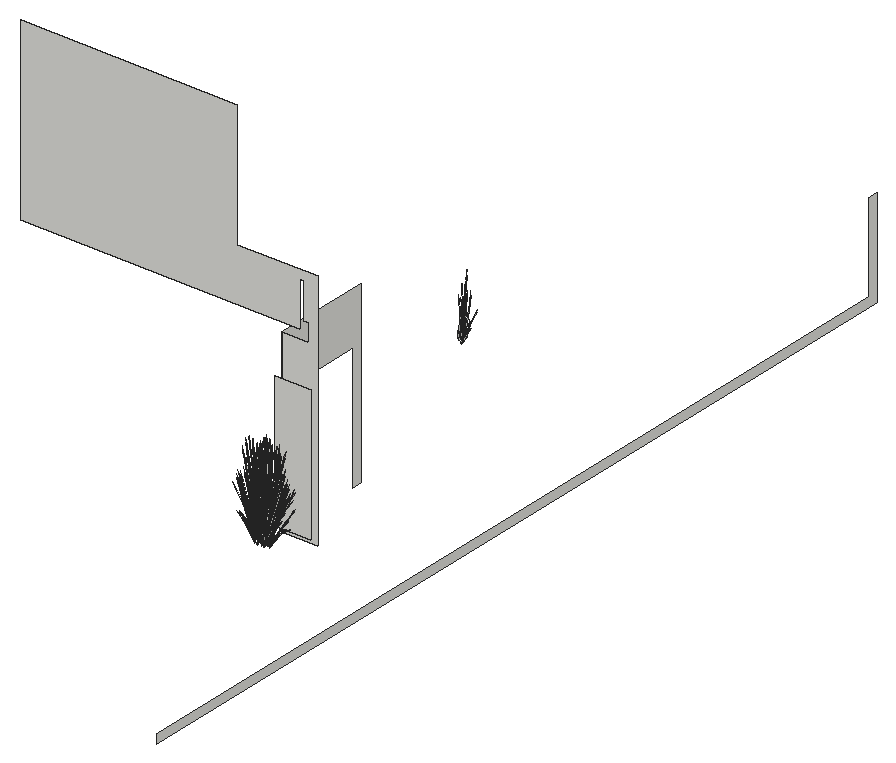
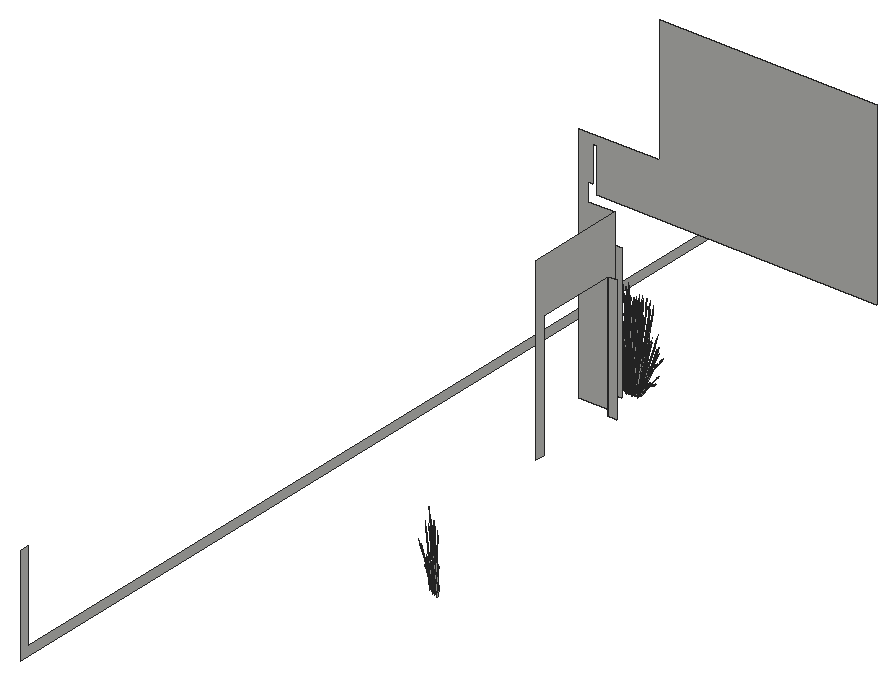
# SketchUp Ruby script. Lengths in inches.
U = 1.inch
M = Sketchup.active_model
def pt(a) = Geom::Point3d.new(a.map { |v| v * U })
def face(e, loops, mat)
  f = e.add_face(loops[0].map { |a| pt(a) })
  loops[1..].each { |l| e.add_face(l.map { |a| pt(a) }).erase! }
  f.material = f.back_material = mat if mat
  f
end
# faces: each face lists its corners as indices into pts; further lists are holes
def faces(e, pts, list, mat = nil) = list.each { |f| face(e, (f[0].is_a?(Array) ? f : [f]).map { |l| l.map { |i| pts[i] } }, mat) }
# xy, xz, yz: faces in a plane at the given z, y or x. An outline is a flat list of corners, or four numbers for a rectangle; further outlines are holes
def ring(l) = l.size == 4 ? [[l[0], l[1]], [l[2], l[1]], [l[2], l[3]], [l[0], l[3]]] : l.each_slice(2).to_a
def flat(e, list, mat, &to3) = list.each { |f| face(e, (f[0].is_a?(Array) ? f : [f]).map { |l| ring(l).map { |u, v| to3.(u, v) } }, mat) }
def xy(e, z, list, mat = nil) = flat(e, list, mat) { |x, y| [x, y, z] }
def xz(e, y, list, mat = nil) = flat(e, list, mat) { |x, z| [x, y, z] }
def yz(e, x, list, mat = nil) = flat(e, list, mat) { |y, z| [x, y, z] }
def lines(e, pts, list) = list.each { |a, b| e.add_line(pt(pts[a]), pt(pts[b])) }
# prism: a flat outline (further loops are holes) pulled along v
def prism(e, loops, v, mat = nil)
  f = face(e, loops, mat); d = Geom::Vector3d.new(v.map { |x| x * U })
  f.pushpull(f.normal.samedirection?(d) ? d.length : -d.length)
end
def box(e, o, s, mat = nil) = prism(e, [[o, [o[0] + s[0], o[1], o[2]], [o[0] + s[0], o[1] + s[1], o[2]], [o[0], o[1] + s[1], o[2]]]], [0, 0, s[2]], mat)
def at(x, y, z, deg = 0) = Geom::Transformation.translation(pt([x, y, z])) * Geom::Transformation.rotation(ORIGIN, Z_AXIS, deg.degrees)
def axes(o, x, y, z) = Geom::Transformation.new([*x, 0, *y, 0, *z, 0, *pt(o).to_a, 1])
def part(name) = M.definitions.add(name)
# library, detail: a bought-in or finely detailed component or shape, given as its bounding box
def library(name, o, s) = part(name).tap { |d| box(d.entities, o, s) }
def detail(e, o, s) = box(e.add_group.entities, o, s)
def put(e, d, t, mat = nil) = e.add_instance(d, t).tap { |i| i.material = mat if mat }
def group(e, t, mat = nil) = e.add_group.tap { |g| g.transformation = t; g.material = mat if mat }.entities
root = M.entities
M.materials.add("LightPink_Translucent").color = [144, 107, 117]
M.materials["LightPink_Translucent"].alpha = 0.75
c1 = part("blade")
p = [[2.15,0.21,22],[0,0.17,0],[0.09,0.45,0],[2.18,0.31,22],[2.29,0.31,22],[0.38,0.45,0],
  [2.48,0.24,33],[2.49,0.24,33],[2.48,0.22,33]]
faces(c1.entities,p,[[0,1,2,3],[4,5,2,3],[6,3,4,7],[8,0,3,6]])
c2 = part("seeds")
p = [[0.3,-0.1,1.38],[-0.01,-0.03,1.59],[-0.01,-0.03,0.03],[0.14,-0.07,-0.07],[0.29,-0.03,3],[0.15,0.01,3.11]]
faces(c2.entities,p,[[0,1,2,3],[1,0,4,5]],"LightPink_Translucent")
c3 = part("blade with seeds")
put(c3.entities,c1,at(0,0,0))
put(c3.entities,c2,axes([2.4,0.25,30.99],[1.5799,-0.05474,1.17369],[-0.12525,1.92788,0.29478],[-0.07173,-0.02425,1.56792]))
xz(root,213,[[342,6,366,96]])
xz(root,219,[[342,0,342,120,360,120,360,132,357,132,357,156,354,156,354,126,166.5,126,166.5,246,312,246,312,162,366,162,366,0]])
xz(root,225,[[336,0,342,84]])
yz(root,342,[[219,0,225,0,225,84,279,84,279,0,285,0,285,120,219,120]])
yz(root,426,[[9,-6,612.89,-6,612.89,60,606.89,60,606.89,0,9,0]])
put(root,c3,axes([340.2,198.67,4.73],[0.25275,-0.59491,0.48003],[0.83094,0.20343,0.3958],[-0.32677,0.03575,0.9933]))
put(root,c3,axes([342.89,198.05,1.59],[-0.88056,0.26122,1.28929],[-0.28027,-0.74951,0.50096],[0.54072,0.01247,1.46642]))
put(root,c3,axes([345.26,198.25,2.62],[0.17258,-0.58229,0.1448],[0.84319,0.10108,-0.41347],[0.15345,0.05979,1.26744]))
put(root,c3,axes([340.14,198.51,4.73],[-0.32857,-0.44488,0.0643],[0.59916,-0.21775,0.50621],[-0.26412,0.04296,0.77189]))
put(root,c3,axes([343.8,199.64,2.36],[1.13071,0.13747,0.45755],[-0.23011,0.77639,0.17955],[-0.16524,-0.07497,1.58856]))
put(root,c3,axes([349.77,199.07,1.49],[-0.04675,-0.09906,1.76342],[0.32428,-0.57943,-0.26939],[0.32711,-0.00833,0.30037]))
put(root,c3,axes([340.12,198.97,1.49],[0.02269,0.10283,1.76342],[-0.45738,0.53699,-0.26939],[-0.32488,-0.02707,0.30037]))
put(root,c3,axes([344.9,198.41,2.72],[-0.53742,-0.54764,0.44739],[0.81403,-0.38564,-0.21531],[0.17391,0.06776,1.43643]))
put(root,c3,axes([342.12,200.91,2.03],[-0.21015,-0.56852,-0.30978],[0.83462,-0.16144,0.30978],[-0.16826,-0.06556,1.38974]))
put(root,c3,axes([343.19,200.875,2.47],[0.96132,-0.17317,0.17642],[0.23737,0.64447,0.35086],[-0.08574,-0.0939,1.60407]))
put(root,c3,axes([345.17,198.44,2.67],[0.90324,-0.43318,-0.29095],[0.60064,0.61207,-0.50002],[0.22285,0.06216,1.59708]))
put(root,c3,axes([348.76,199.58,4.53],[0.74348,0.18202,-0.35414],[-0.21685,0.53102,0.4572],[0.29933,-0.04869,0.87481]))
put(root,c3,axes([341.89,201.15,2.02],[-0.83726,-0.32623,-0.49651],[0.50045,-0.58498,0],[-0.19069,-0.0743,1.57504]))
put(root,c3,axes([347.45,197.29,2.02],[0.83726,0.32623,-0.49651],[-0.50045,0.58498,0],[0.19069,0.0743,1.57504]))
put(root,c3,axes([340.03,198.74,4.53],[-0.74348,-0.18202,-0.35414],[0.21685,-0.53102,0.4572],[-0.29933,0.04869,0.87481]))
put(root,c3,axes([345.86,199.15,2.21],[1.00089,0,0],[0,0.67548,0],[0,0,1.78407]))
put(root,c3,axes([344.17,200,2.67],[-0.90324,0.43318,-0.29095],[-0.60064,-0.61207,-0.50002],[-0.22285,-0.06216,1.59708]))
put(root,c3,axes([346.15,197.57,2.47],[-0.96132,0.17317,0.17642],[-0.23737,-0.64447,0.35086],[0.08574,0.0939,1.60407]))
put(root,c3,axes([346.74,198.93,3.875],[-0.37107,0.01478,1.71376],[0.24616,-0.64047,0.13857],[0.5288,0.03961,0.73262]))
put(root,c3,axes([347.22,197.53,2.03],[0.21015,0.56852,-0.30978],[-0.83462,0.16144,0.30978],[0.16826,0.06556,1.38974]))
put(root,c3,axes([348.66,199.81,4.73],[0.32857,0.44488,0.0643],[-0.59916,0.21775,0.50621],[0.26412,-0.04296,0.77189]))
put(root,c3,axes([345.54,198.81,2.38],[-1.13071,-0.13747,0.49198],[0.23011,-0.77639,0.19306],[0.16524,0.07497,1.70813]))
put(root,c3,axes([348.59,199.65,4.73],[-0.25275,0.59491,0.48003],[-0.83094,-0.20343,0.3958],[0.32677,-0.03575,0.9933]))
put(root,c3,axes([344.64,200.72,2.2],[-0.29189,-0.56252,0],[0.83351,-0.19699,0],[0,0,1.54371]))
put(root,c3,axes([344.08,200.19,2.62],[-0.17258,0.58229,0.1448],[-0.84319,-0.10108,-0.41347],[-0.15345,-0.05979,1.26744]))
put(root,c3,axes([340.81,198.68,5.05],[0.74348,0.18202,0.35414],[-0.21685,0.53102,-0.4572],[-0.29933,0.04869,0.87481]))
put(root,c3,axes([345.73,200.64,2.18],[0.93921,-0.22138,-0.19198],[0.33003,0.6377,0.00008],[0.10367,-0.02447,1.73897]))
put(root,c3,axes([346.05,200.91,2.47],[0.25843,-0.64844,0.17642],[0.9457,0.1835,0.35086],[-0.16336,0.00316,1.60407]))
put(root,c3,axes([345.84,199.44,2.21],[0.62448,0.42144,0],[-0.62448,0.42144,0],[0,0,1.69266]))
put(root,c3,axes([342.29,198.65,3.34],[0.25429,-0.09438,1.77064],[0.08769,0.65901,0.13857],[-0.5508,0.08745,0.63284]))
put(root,c3,axes([347.53,199.26,2.47],[-0.70288,-0.47526,0.17642],[0.70832,-0.46097,0.35086],[-0.07763,0.09706,1.60407]))
put(root,c3,axes([346.23,198.54,2.06],[0.9306,0.10697,-0.62353],[-0.19638,0.65984,-0.16365],[0.27771,0.07995,1.37633]))
put(root,c3,axes([350.34,199.69,2.77],[-0.55274,0.10771,1.1486],[0.26018,-0.44517,0.84392],[0.29323,0.03046,0.25299]))
put(root,c3,axes([344.43,200.98,2.2],[-0.90188,-0.29293,0],[0.43405,-0.60866,0],[0,0,1.62707]))
put(root,c3,axes([345.18,200.2,2.46],[-0.87356,-0.52515,-0.25192],[0.73507,-0.5897,0.5513],[-0.23523,0.06143,1.68216]))
put(root,c3,axes([342.88,201.2,2.48],[0.83726,0.32623,0.49651],[-0.50045,0.58498,0],[-0.19069,-0.0743,1.57504]))
put(root,c3,axes([345.83,198.95,2.72],[0.43405,-0.58792,0.44739],[0.90188,0.28295,-0.21531],[0,0.13553,1.43643]))
put(root,c3,axes([350.09,201.57,4.71],[-0.08089,-0.05712,1.77383],[0.17695,-0.61228,-0.16761],[0.31864,-0.03912,0.31391]))
put(root,c3,axes([339.56,199.09,4.72],[-0.14609,0.08471,1.74944],[0.01243,0.61893,-0.27667],[-0.33486,0.08049,0.14031]))
put(root,c3,axes([345.67,199.28,2.29],[0,0.75458,-0.05637],[-1.11865,0,0],[0,0.02371,1.79368]))
put(root,c3,axes([340.54,199.01,4.68],[-0.24236,0.59349,-0.51099],[-0.83094,-0.20343,-0.3958],[-0.33455,0.05442,0.97773]))
put(root,c3,axes([340.5,198.5,5.03],[0.45012,0.59081,-0.1216],[-0.79888,0.29033,-0.67495],[-0.33665,0.07795,1.02557]))
put(root,c3,axes([345.75,198.75,2.21],[0.53742,0.54764,-0.44739],[-0.81403,0.38564,0.21531],[0.17391,0.06776,1.43643]))
put(root,c3,axes([349.38,201.0625,3.93],[-0.17122,-0.54847,-0.03492],[0.80929,-0.12609,-0.15832],[0.169,0.03477,0.52218]))
put(root,c3,axes([342.4,201.55,2.375],[-0.55932,0.6538,0],[-0.93577,-0.36461,-0.51607],[-0.21313,-0.08304,1.63711]))
put(root,c3,axes([347.28,201.05,5.03],[0.0479,-0.66354,-0.1216],[0.90696,0.01814,-0.67495],[0.3493,0.04609,1.02557]))
put(root,c3,axes([348.11,199.27,2.48],[0,-0.65246,0.49651],[1.00089,0,0],[0,0.1486,1.57504]))
put(root,c3,axes([345.6,199.76,2.72],[0.97146,-0.04028,0.44739],[0.08785,0.66859,-0.21531],[-0.17391,0.06776,1.43643]))
put(root,c3,axes([346.21,199.08,2.62],[0.83351,-0.19028,0.1448],[0.29189,0.54335,-0.41347],[0,0.11958,1.26744]))
put(root,c3,axes([347.14,200.79,5.05],[-0.50902,-0.40851,0.35414],[0.58122,-0.38671,-0.4572],[0.29531,0.05884,0.87481]))
put(root,c3,axes([344.74,200.09,2.21],[-0.97146,0.04028,-0.44739],[-0.08785,-0.66859,0.21531],[-0.17391,0.06776,1.43643]))
put(root,c3,axes([349.31,200.41,2.59],[-0.21545,-0.16047,1.43002],[0.28033,-0.53085,-0.30754],[0.43591,0.07191,0.61141]))
put(root,c3,axes([345.45,200.99,2.2],[0.90188,0.29293,0],[-0.43405,0.60866,0],[0,0,1.74954]))
put(root,c3,axes([348.07,200.65,4.72],[0.19191,-0.01103,1.74944],[0.52639,-0.5069,-0.27667],[0.34136,0.06691,0.14031]))
put(root,c3,axes([345.8125,201.64,2.19],[-0.55235,-0.65609,-0.05142],[0.93577,-0.36461,0.51607],[-0.23059,0.06247,1.6363]))
put(root,c3,axes([345.62,200.05,2.62],[0.66093,0.39201,0.1448],[-0.5513,0.44227,-0.41347],[-0.15345,0.05979,1.26744]))
put(root,c3,axes([340.4,200.15,4.73],[-0.22187,-0.60049,0.48003],[0.87033,-0.10422,0.3958],[-0.25651,0.14123,0.9933]))
put(root,c3,axes([340.23,200.04,4.73],[-0.61415,-0.2744,0.0643],[0.35756,-0.39076,0.50621],[-0.1969,0.12633,0.77189]))
put(root,c3,axes([340.51,199.3125,3.875],[0.31041,-0.13801,1.71376],[0.26133,0.63772,0.13857],[-0.48731,0.14413,0.73262]))
put(root,c3,axes([347.33,200.73,4.98],[0.89428,0.01571,-0.71045],[-0.06006,0.66153,0.08574],[0.37886,0.06981,1.00501]))
put(root,c3,axes([346.32,201.26,2.48],[0.83726,-0.32623,0.49651],[0.50045,0.58498,0],[-0.19069,0.0743,1.57504]))
put(root,c3,axes([345.13,200.74,2.29],[0.38895,0.74956,-0.06012],[-1.11135,0.26265,0],[0.01358,0.02618,1.72173]))
put(root,c3,axes([345.5625,201.55,2.03],[-0.83462,-0.16144,-0.30978],[0.21015,-0.56852,0.30978],[-0.16826,0.06556,1.38974]))
put(root,c3,axes([339.54,200.4,2.59],[0.3109,0.05356,1.43002],[0.20038,0.54709,-0.30754],[-0.42231,0.10241,0.61141]))
put(root,c3,axes([340.93,199.95,5.05],[0.77872,-0.09325,0.35414],[0.20563,0.53305,-0.4572],[-0.22316,0.14318,0.87481]))
put(root,c3,axes([348.79,199.39,2.375],[1.11865,0,0],[0,0.72922,-0.51607],[0,0.16609,1.63711]))
put(root,c3,axes([337.93,199.72,4.71],[0.11417,0.0175,1.77383],[0.35319,0.57649,-0.16761],[-0.23371,0.15131,0.31391]))
put(root,c3,axes([348.34,199.76,2.2],[-1.1181,-0.00522,-0.04976],[0,-0.72922,0.49943],[-0.03514,0.166,1.58352]))
put(root,c3,axes([345.92,199.125,2.67],[1.00749,0.31132,-0.29095],[-0.48511,0.65709,-0.50002],[0.03166,0.16133,1.59708]))
put(root,c3,axes([338.89,201.55,2.77],[0.37283,-0.29571,1.1486],[0.14711,0.46813,0.84392],[-0.26943,0.08382,0.25299]))
put(root,c3,axes([347.87,201,4.53],[0.50902,0.40851,-0.35414],[-0.58122,0.38671,0.4572],[0.29531,0.05884,0.87481]))
put(root,c3,axes([348.11,199.87,2.03],[-0.62448,0.40708,-0.30978],[-0.62448,-0.40708,0.30978],[0,0.13112,1.38974]))
put(root,c3,axes([345.42,199.91,2.67],[0.10425,0.7445,-0.29095],[-1.08575,0.04502,-0.50002],[-0.19119,0.09917,1.59708]))
put(root,c3,axes([347.61,201.16,4.73],[-0.04505,0.49615,0.0643],[-0.68022,-0.0136,0.50621],[0.26056,0.05192,0.77189]))
put(root,c3,axes([345.81,199.61,2.21],[-0.43405,0.58792,-0.44739],[-0.90188,-0.28295,0.21531],[0,0.13553,1.43643]))
put(root,c3,axes([340.3,200.27,4.53],[-0.77872,0.09325,-0.35414],[-0.20563,-0.53305,0.4572],[-0.22316,0.14318,0.87481]))
put(root,c3,axes([347.67,201,4.73],[-0.65964,0.42992,0.48003],[-0.5689,-0.45657,0.3958],[0.30948,0.0793,0.9933]))
put(root,c3,axes([339.17,201.47,5.65],[0.78943,0.17416,-0.06488],[-0.24284,0.53604,-0.29416],[-0.12912,0.08139,0.97024]))
put(root,c3,axes([344.77,200.47,2.06],[-0.60257,0.49041,-0.62353],[-0.74854,-0.44469,-0.16365],[-0.24146,0.12234,1.37633]))
put(root,c3,axes([345.57,201.5,5.05],[-0.13817,-0.52554,0.35414],[0.78985,-0.13877,-0.4572],[0.21215,0.1506,0.87481]))
put(root,c3,axes([345.84,201.3,2.33],[1.11998,0.21207,0.30756],[-0.2802,0.75803,-0.36492],[-0.18537,0.09487,1.64885]))
put(root,c3,axes([345.76,201.8125,2.02],[-0.83726,0.32623,-0.49651],[-0.50045,-0.58498,0],[-0.19069,0.0743,1.57504]))
put(root,c3,axes([348.54,199.88,2.02],[0,0.65246,-0.49651],[-1.00089,0,0],[0,0.1486,1.57504]))
put(root,c3,axes([346.04,199.95,3.875],[-0.3323,-0.11241,1.71376],[0.68769,-0.4716,0.13857],[0.42861,0.21275,0.73262]))
put(root,c3,axes([346.1,198.47,4.47],[-0.77304,-0.33901,1.38283],[0.81626,-0.52782,0.59665],[0.24941,0.31809,1.33663]))
put(root,c3,axes([340.53,199.9,5.03],[0.82753,0.35977,-0.1216],[-0.47675,0.52101,-0.67495],[-0.2338,0.18111,1.02557]))
put(root,c3,axes([347.27,201.23,2.77],[-0.5037,-0.18761,1.1486],[0.6504,-0.19062,0.84392],[0.17543,0.16147,0.25299]))
put(root,c3,axes([345.5,201.77,5.03],[0.53309,-0.55848,-0.1216],[0.77201,0.32175,-0.67495],[0.26836,0.15779,1.02557]))
put(root,c3,axes([341.64,199.74,3.875],[0.22344,-0.20048,1.71376],[0.56419,0.54113,0.13857],[-0.38697,0.24643,0.73262]))
put(root,c3,axes([340.94,200.33,4.68],[0.22982,0.59576,-0.51099],[-0.87033,0.10422,-0.3958],[-0.24941,0.16002,0.97773]))
put(root,c3,axes([341.98,201.02,5.05],[0.60531,-0.34352,0.35414],[0.573,0.39225,-0.4572],[-0.08718,0.19929,0.87481]))
put(root,c3,axes([346.52,201.71,2.375],[0.55932,0.6538,0],[-0.93577,0.36461,-0.51607],[-0.21313,0.08304,1.63711]))
put(root,c3,axes([344.8,202.23,4.71],[0.00265,-0.07899,1.77383],[0.76665,-0.34851,-0.16761],[0.2663,0.12439,0.31391]))
put(root,c3,axes([347.41,201.93,1.49],[0.06518,-0.0942,1.76342],[0.82057,-0.27742,-0.26939],[0.24877,0.14358,0.30037]))
put(root,c3,axes([346.04,199.12,2.84],[-0.02444,-0.61432,1.41272],[1.10603,0.15924,0.59816],[-0.26159,0.33615,1.3335]))
put(root,c3,axes([346.33,199.79,2.09],[0.32803,0.59738,-0.69212],[-0.94492,0.21515,-0.18165],[0.03626,0.20229,1.52773]))
put(root,c3,axes([341.4375,201.33,4.73],[-0.73517,-0.0304,0.0643],[0.02016,-0.45906,0.50621],[-0.07693,0.17585,0.77189]))
put(root,c3,axes([339.875,201.85,1.49],[0.12,0.06519,1.76342],[0.20347,0.60397,-0.26939],[-0.26596,0.12879,0.30037]))
put(root,c3,axes([341.67,201.37,4.73],[-0.63704,-0.44518,0.48003],[0.67652,-0.38394,0.3958],[-0.11751,0.20886,0.9933]))
put(root,c3,axes([346.13,201.49,4.68],[0.88277,-0.1551,-0.51099],[0.15442,0.58737,-0.3958],[0.23711,0.16832,0.97773]))
put(root,c3,axes([343.68,201.58,5.05],[0.2697,-0.50175,0.35414],[0.78684,0.14635,-0.4572],[0.07215,0.20201,0.87481]))
put(root,c3,axes([347.35,202.09,2.67],[-0.57368,-0.02046,1.0506],[0.37886,-0.43461,0.58006],[0.22663,0.15441,0.8241]))
put(root,c3,axes([345.7,201.97,4.73],[-0.4066,0.41448,0.0643],[-0.57901,-0.24131,0.50621],[0.18719,0.13288,0.77189]))
put(root,c3,axes([344.74,203.37,5.65],[0.61821,-0.37431,-0.06488],[0.56645,0.40995,-0.29416],[0.03988,0.11616,0.97024]))
put(root,c3,axes([345.87,201.86,4.73],[-0.88979,0.14973,0.48003],[-0.15442,-0.58737,0.3958],[0.20926,0.17311,0.9933]))
put(root,c3,axes([341.48,200.24,3.875],[0.16657,-0.22426,1.71376],[0.69879,0.4641,0.13857],[-0.31524,0.28926,0.73262]))
put(root,c3,axes([345.48,201.03,2.59],[0.01579,-0.21629,1.43002],[0.75442,-0.24159,-0.30754],[0.23289,0.25887,0.61141]))
put(root,c3,axes([343.4375,202.04,4.73],[-0.6592,0.22175,0.0643],[-0.32265,-0.40436,0.50621],[0.06366,0.17825,0.77189]))
put(root,c3,axes([341.67,201.5,4.53],[-0.60531,0.34352,-0.35414],[-0.573,-0.39225,0.4572],[-0.08718,0.19929,0.87481]))
put(root,c3,axes([339.58,201.4,4.72],[-0.02224,0.12912,1.74944],[0.63107,0.44917,-0.27667],[-0.16521,0.21241,0.14031]))
put(root,c3,axes([341.6,201.11,5.4],[0.98321,0.03233,-0.13498],[-0.02687,0.61208,-0.74919],[-0.0683,0.23574,1.13838]))
put(root,c3,axes([343.42,201.79,5.03],[0.87543,-0.30377,-0.1216],[0.4302,0.53915,-0.67495],[0.1155,0.2272,1.02557]))
put(root,c3,axes([343.67,201.99,5.0625],[-0.88151,-0.17057,0.53283],[0.30143,-0.56078,0.43934],[0.05297,0.22053,1.10256]))
put(root,c3,axes([342.05,202.84,2.77],[-0.02315,-0.38796,1.1486],[0.57853,0.27671,0.84392],[-0.11378,0.18492,0.25299]))
put(root,c3,axes([343.58,201.91,1.49],[0.14478,-0.0355,1.76342],[0.8709,0.19542,-0.26939],[0.02547,0.22025,0.30037]))
put(root,c3,axes([342.27,201.34,5],[0.64041,0.4384,-0.5672],[-0.67652,0.38394,-0.43934],[-0.09744,0.22274,1.08528]))
put(root,c3,axes([341.57,202,2.82],[0.8127,-0.11554,0.06507],[0.18684,0.46549,-0.86304],[-0.05152,0.23564,0.7736]))
put(root,c3,axes([344.17,201.77,4.68],[0.87941,0.16356,-0.51099],[-0.30143,0.56078,-0.3958],[0.08064,0.22578,0.97773]))
put(root,c3,axes([344.67,200.61,3.875],[-0.2045,-0.20949,1.71376],[0.94495,-0.17636,0.13857],[0.21357,0.32887,0.73262]))
put(root,c3,axes([343.77,202.11,4.53],[-0.2697,0.50175,-0.35414],[-0.78684,-0.14635,0.4572],[0.07215,0.20201,0.87481]))
put(root,c3,axes([342.07,201.14,5.34],[-0.02328,0.60353,-0.7886],[-0.98022,-0.04053,0.09517],[-0.10344,0.25568,1.11556]))
put(root,c3,axes([339.51,202.72,4.71],[0.10149,-0.03939,1.77383],[0.83886,0.26202,-0.16761],[-0.01971,0.21816,0.31391]))
put(root,c3,axes([343,200.71,3.875],[-0.0219,-0.25042,1.71376],[0.94901,0.16613,0.13857],[-0.0587,0.35688,0.73262]))
put(root,c3,axes([343.85,201.66,4.98],[0.42698,0.53052,-0.71045],[-0.87893,0.29566,0.08574],[0.09984,0.25633,1.00501]))
put(root,c3,axes([341.38,202.49,2.59],[0.28231,-0.10293,1.43002],[0.69701,0.31035,-0.30754],[-0.20746,0.26854,0.61141]))
put(root,c3,axes([343.21,203,4.72],[0.1134,0.10507,1.74944],[0.91515,0.04128,-0.27667],[0.09203,0.23172,0.14031]))
put(root,c3,axes([341.74,201.99,3.36],[0.01966,-0.33682,1.54345],[0.88405,0.17791,0.21329],[-0.0766,0.35897,0.72882]))
put(root,c3,axes([291.92,432.65,4.72],[-0.00864,-0.12985,1.74944],[-0.72937,-0.3753,-0.27667],[0.11277,-0.2275,0.14031]))
put(root,c3,axes([289.45,433.28,3.875],[-0.16657,0.22426,1.71376],[-0.69879,-0.4641,0.13857],[0.31524,-0.28926,0.73262]))
put(root,c3,axes([290.96,433.23,4.53],[0.60531,-0.34352,-0.35414],[0.573,0.39225,0.4572],[0.08718,-0.19929,0.87481]))
put(root,c3,axes([291.71,433.02,1.49],[-0.1339,-0.0514,1.76342],[-0.34394,-0.57425,-0.26939],[0.23202,-0.15583,0.30037]))
put(root,c3,axes([290.96,433.36,4.73],[0.63704,0.44518,0.48003],[-0.67652,0.38394,0.3958],[0.11751,-0.20886,0.9933]))
put(root,c3,axes([291.19,433.4,4.73],[0.73517,0.0304,0.0643],[-0.02016,0.45906,0.50621],[0.07693,-0.17585,0.77189]))
put(root,c3,axes([291.71,434.64,4.98],[0.4673,-0.51481,-0.71045],[0.81887,0.36587,0.08574],[0.27902,-0.18652,1.00501]))
put(root,c3,axes([291.69,434.4,4.68],[-0.22982,-0.59576,-0.51099],[0.87033,-0.10422,-0.3958],[0.24941,-0.16002,0.97773]))
put(root,c3,axes([292.1,434.82,5.03],[-0.82753,-0.35977,-0.1216],[0.47675,-0.52101,-0.67495],[0.2338,-0.18111,1.02557]))
put(root,c3,axes([292.39,434.16,2.59],[-0.31959,-0.01933,1.43002],[-0.32741,-0.51843,-0.30754],[0.39262,-0.14666,0.61141]))
put(root,c3,axes([294.13,434.67,4.71],[-0.11685,-0.00496,1.77383],[-0.48522,-0.53096,-0.16761],[0.19486,-0.17458,0.31391]))
put(root,c3,axes([288.41,434.375,2.06],[0.60257,-0.49041,-0.62353],[0.74854,0.44469,-0.16365],[0.24146,-0.12234,1.37633]))
put(root,c3,axes([292.75,433.21,2.77],[-0.29798,0.33213,1.1486],[-0.25612,-0.44624,0.84392],[0.24611,-0.11182,0.25299]))
